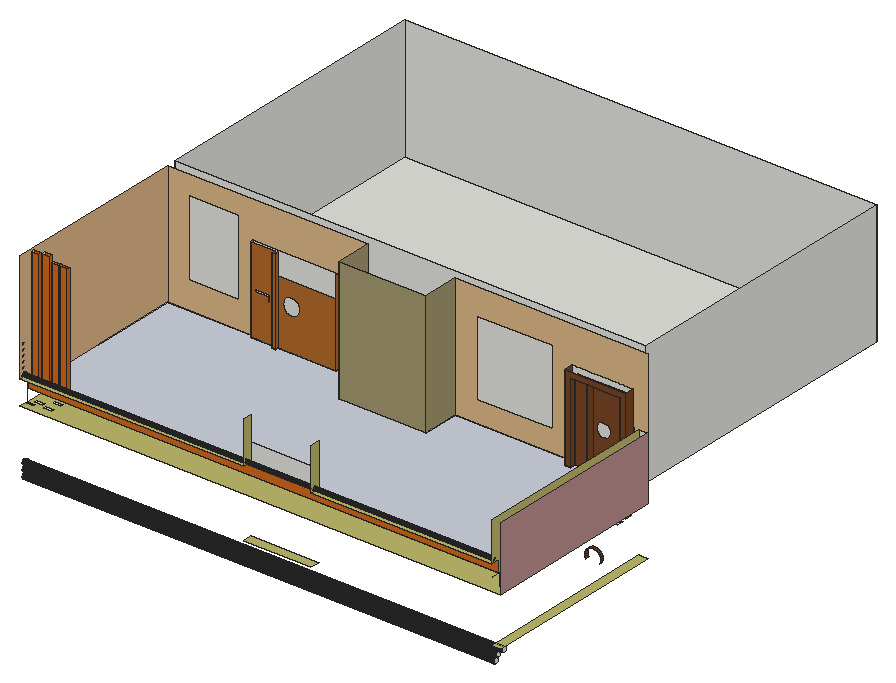
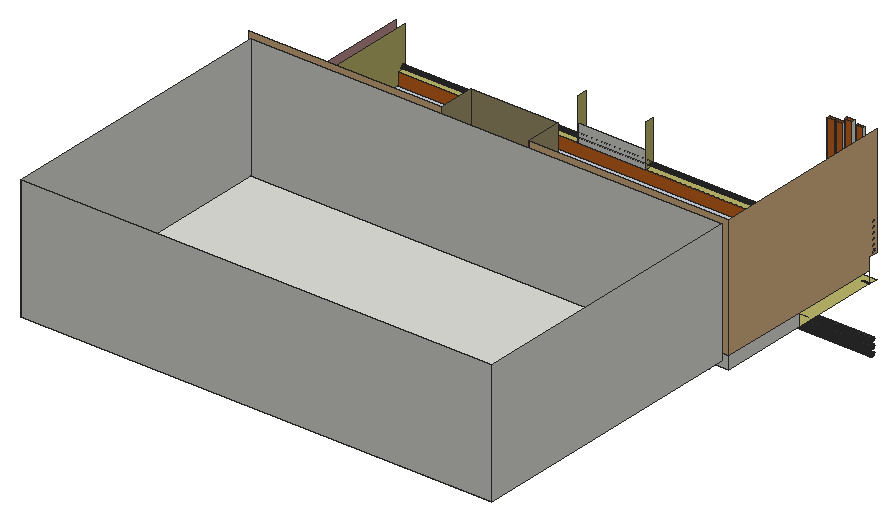
# SketchUp Ruby script. Lengths in inches.
U = 1.inch
M = Sketchup.active_model
def pt(a) = Geom::Point3d.new(a.map { |v| v * U })
def face(e, loops, mat)
  f = e.add_face(loops[0].map { |a| pt(a) })
  loops[1..].each { |l| e.add_face(l.map { |a| pt(a) }).erase! }
  f.material = f.back_material = mat if mat
  f
end
# faces: each face lists its corners as indices into pts; further lists are holes
def faces(e, pts, list, mat = nil) = list.each { |f| face(e, (f[0].is_a?(Array) ? f : [f]).map { |l| l.map { |i| pts[i] } }, mat) }
# xy, xz, yz: faces in a plane at the given z, y or x. An outline is a flat list of corners, or four numbers for a rectangle; further outlines are holes
def ring(l) = l.size == 4 ? [[l[0], l[1]], [l[2], l[1]], [l[2], l[3]], [l[0], l[3]]] : l.each_slice(2).to_a
def flat(e, list, mat, &to3) = list.each { |f| face(e, (f[0].is_a?(Array) ? f : [f]).map { |l| ring(l).map { |u, v| to3.(u, v) } }, mat) }
def xy(e, z, list, mat = nil) = flat(e, list, mat) { |x, y| [x, y, z] }
def xz(e, y, list, mat = nil) = flat(e, list, mat) { |x, z| [x, y, z] }
def yz(e, x, list, mat = nil) = flat(e, list, mat) { |y, z| [x, y, z] }
def lines(e, pts, list) = list.each { |a, b| e.add_line(pt(pts[a]), pt(pts[b])) }
# prism: a flat outline (further loops are holes) pulled along v
def prism(e, loops, v, mat = nil)
  f = face(e, loops, mat); d = Geom::Vector3d.new(v.map { |x| x * U })
  f.pushpull(f.normal.samedirection?(d) ? d.length : -d.length)
end
def box(e, o, s, mat = nil) = prism(e, [[o, [o[0] + s[0], o[1], o[2]], [o[0] + s[0], o[1] + s[1], o[2]], [o[0], o[1] + s[1], o[2]]]], [0, 0, s[2]], mat)
def at(x, y, z, deg = 0) = Geom::Transformation.translation(pt([x, y, z])) * Geom::Transformation.rotation(ORIGIN, Z_AXIS, deg.degrees)
def axes(o, x, y, z) = Geom::Transformation.new([*x, 0, *y, 0, *z, 0, *pt(o).to_a, 1])
def part(name) = M.definitions.add(name)
# library, detail: a bought-in or finely detailed component or shape, given as its bounding box
def library(name, o, s) = part(name).tap { |d| box(d.entities, o, s) }
def detail(e, o, s) = box(e.add_group.entities, o, s)
def put(e, d, t, mat = nil) = e.add_instance(d, t).tap { |i| i.material = mat if mat }
def group(e, t, mat = nil) = e.add_group.tap { |g| g.transformation = t; g.material = mat if mat }.entities
root = M.entities
M.materials.add("[0036_BurlyWood]").color = [222, 184, 135]
M.materials.add("[0041_Chocolate]").color = [210, 105, 30]
M.materials.add("[0057_DarkKhaki]").color = [189, 183, 107]
M.materials.add("[0119_RosyBrown]").color = [188, 143, 143]
M.materials.add("[Marble Carrara Floor Tile]").color = [204, 208, 219]
M.materials.add("[Sandstone]").color = [118, 81, 52]
M.materials.add("[Wood Bamboo]").color = [177, 105, 43]
M.materials.add("[Wood Floor Parquet]").color = [145, 89, 39]
M.materials.add("[Wood Lumber ButtJoined]").color = [164, 152, 112]
M.materials.add("[Wood Veneer 01]").color = [120, 70, 37]
xy(root,289,[[115.45,186.3,116.7,189.3]],"[Wood Bamboo]")
xy(root,292.0625,[[105.14,186.3,115.45,189.3]],"[Wood Bamboo]")
xy(root,293.5,[[105.14,186.3,116.7,189.3]],"[Wood Bamboo]")
xy(root,300,[[471,12,480,192.3]],"[0057_DarkKhaki]")
xy(root,306.625,[[227.54,12,293.97,21]],"[0057_DarkKhaki]")
xy(root,308.5,[[130.66,186.3,176.72,189.3]],"[Wood Bamboo]")
xy(root,320.5625,[[130.66,186.3,176.72,189.3]],"[Wood Bamboo]")
xy(root,324,[[395.16,186.3,410.94,189.3],[410.94,186.3,411.65,189.3],[411.65,186.3,455.16,189.3],[395.16,189.3,455.16,192.3]])
xy(root,324,[[120.23,186.3,123.15,189.3],[100.9,189.3,184.9,192.3]],"[Wood Bamboo]")
xy(root,331.9375,[[387.22,186.3,463.09,192.3]],"[Wood Veneer 01]")
xy(root,335.94,[[309.99,189.3,343.2,192.3],[347.01,189.3,376.42,192.3]])
xy(root,340.15,[[30.47,189.3,55.47,192.3],[60.04,189.3,80.47,192.3]],"[Wood Floor Parquet]")
xy(root,340.75,[[305.18,189.3,381.23,192.3]],"[Wood Floor Parquet]")
xy(root,344.59,[[26.03,189.3,84.9,192.3]],"[Wood Floor Parquet]")
xy(root,348,[[9,12,9,18.8125,16.75,18.8125,16.75,21,9,21,9,192.3,92.74,192.3,92.74,189.3,116.27,189.3,116.27,186.3,119.49,186.3,119.49,189.3,176.74,189.3,176.74,192.3,205.37,192.3,205.37,156.87,290.8125,156.87,290.8125,192.3,405.34,192.3,405.34,183.3,410.93,183.3,410.93,189.3,426.75,189.3,426.75,183.3,427.96,183.3,427.96,189.3,459.74,189.3,459.74,183.3,465.34,183.3,465.34,192.3,480,192.3,480,12]],"[0057_DarkKhaki]")
xy(root,349.8125,[[26.9375,18.8125,34.6875,21]])
xy(root,351.875,[[17.75,18.8125,25.5,21]])
xy(root,357.3125,[[35.9375,18.8125,43.6875,21]])
xy(root,360,[[471,21,471.0625,192.3],[405.34,183.3,410.93,192.3],[426.75,183.3,427.96,183.3,427.96,189.3,459.74,189.3,459.74,192.3,410.93,192.3,410.93,189.3,426.75,189.3],[459.74,183.3,465.34,192.3],[116.27,186.3,119.49,186.3,119.49,189.3,176.74,189.3,176.74,192.3,92.74,192.3,92.74,189.3,116.27,189.3],
  [9,201.23,471,483]])
xy(root,360,[[9,21,471,21,471,192.3,465.34,192.3,465.34,183.3,459.74,183.3,459.74,189.3,427.96,189.3,427.96,183.3,426.75,183.3,426.75,189.3,410.93,189.3,410.93,183.3,405.34,183.3,405.34,192.3,290.8125,192.3,290.8125,156.87,205.37,156.87,205.37,192.3,176.74,192.3,176.74,189.3,119.49,189.3,119.49,186.3,116.27,186.3,116.27,189.3,92.74,189.3,92.74,192.3,9,192.3]],"[Marble Carrara Floor Tile]")
xy(root,372,[[9,12,227.54,12,227.54,21,50.08,21,50.08,18,42.9,18,42.9,21,41.83,21,41.83,18,34.65,18,34.65,21,32.83,21,32.83,18,25.65,18,25.65,21,22.21,21,22.21,18,15.02,18,15.02,21,9,21],[293.97,12,471.0625,21]],"[0057_DarkKhaki]")
xz(root,18,[[15.02,372,22.21,483.12],[25.65,372,32.83,485],[34.65,372,41.83,479.9375],[42.9,372,50.08,480]],"[0041_Chocolate]")
xz(root,21,[[227.54,372,293.97,389.38]])
xz(root,21,[[9,360,9,372,15.02,372,15.02,483.12,22.21,483.12,22.21,372,25.65,372,25.65,485,32.83,485,32.83,372,34.65,372,34.65,479.9375,41.83,479.9375,41.83,372,42.9,372,42.9,480,50.08,480,50.08,372,471.0625,372,471.0625,360]],"[0041_Chocolate]")
xz(root,156.87,[[205.37,348,290.8125,360]])
xz(root,156.87,[[205.37,360,290.8125,480]],"[Wood Lumber ButtJoined]")
xz(root,183.3,[[405.34,348,410.93,360],[426.75,348,427.96,360],[459.74,348,465.34,360]])
xz(root,183.3,[[405.34,360,410.93,360,410.93,438.4,459.74,438.4,459.74,360,465.34,360,465.34,444,405.34,444],[426.75,360,427.96,438.4]],"[Wood Veneer 01]")
xz(root,186.3,[[116.27,348,119.49,360]])
xz(root,186.3,[[115.45,289,116.7,289,116.7,293.5,105.14,293.5,105.14,292.0625,115.45,292.0625],[130.66,308.5,176.72,320.5625],[116.27,360,119.49,444]],"[Wood Bamboo]")
xz(root,189.3,[[115.45,289,115.45,292.0625,105.14,292.0625,105.14,293.5,116.7,293.5,116.7,289],[130.66,308.5,176.72,320.5625],[92.74,348,116.27,360],[119.49,348,176.74,360],[410.93,348,426.75,360],
  [427.96,348,459.74,360]])
xz(root,189.3,[[[123.15,303.1875,184.9,324],[130.66,308.5,176.72,320.5625]],[[92.74,360,116.27,444],[109.64,396.16,109.64,401.1,96.64,401.1,96.64,403.6,111.7,403.6,111.7,396.16]],[[119.49,360,176.74,422.86],[132.85,392.25,130.72,392.53,128.73,393.36,127.02,394.67,125.71,396.38,124.88,398.37,124.6,400.5,124.88,402.64,125.71,404.63,127.02,406.34,128.73,407.65,130.72,408.47,132.85,408.75,134.99,408.47,136.98,407.65,138.68,406.34,140,404.63,140.82,402.64,141.1,400.5,140.82,398.37,140,396.38,138.68,394.67,136.98,393.36,134.99,392.53]]],"[Wood Bamboo]")
xz(root,189.3,[[410.93,360,426.75,438.4],[[427.96,360,459.74,438.4],[438.92,392.76,437.13,393,435.46,393.69,434.02,394.8,432.92,396.23,432.22,397.91,431.99,399.7,432.22,401.5,432.92,403.17,434.02,404.61,435.46,405.71,437.13,406.4,438.92,406.64,440.72,406.4,442.39,405.71,443.83,404.61,444.93,403.17,445.625,401.5,445.86,399.7,445.625,397.91,444.93,396.23,443.83,394.8,442.39,393.69,440.72,393]]],"[Wood Veneer 01]")
xz(root,192.3,[[9,348,92.74,360],[176.74,348,205.37,360],[290.8125,348,405.34,360],[465.34,348,466.21,360],[466.21,348,471,360],
  [471,348,480,360],[405.34,360,405.34,444,465.34,444,465.34,360,459.74,360,459.74,438.4,410.93,438.4,410.93,360],[471.0625,360,480,396]])
xz(root,192.3,[[[9,360,92.74,360,92.74,444,176.74,444,176.74,360,205.37,360,205.37,480,9,480],[29.8125,386.98,79,461.6]],[[290.8125,360,405.34,360,405.34,444,465.34,444,465.34,360,471.0625,360,471.0625,410.4375,480,410.4375,480,480,290.8125,480],[312.25,380.84,386.1875,454.78]]],"[0036_BurlyWood]")
xz(root,201.23,[[9,360,471,480]])
xz(root,483,[[9,360,471,480]])
yz(root,9,[[106.65,348,192.3,360],[201.23,360,483,480],[15.36,372.95,14.91,373.01,14.49,373.1875,14.125,373.47,13.85,373.83,13.67,374.25,13.61,374.7,13.67,375.16,13.85,375.58,14.125,375.94,14.49,376.22,14.91,376.39,15.36,376.45,15.82,376.39,16.24,376.22,16.6,375.94,16.88,375.58,17.05,375.16,17.11,374.7,17.05,374.25,16.88,373.83,16.6,373.47,16.24,373.1875,15.82,373.01]])
yz(root,9,[[[21,360,192.3,360,192.3,480,12,480,12,372,21,372],[15.36,399.52,14.91,399.58,14.49,399.75,14.125,400.03,13.85,400.39,13.67,400.8125,13.61,401.27,13.67,401.72,13.85,402.14,14.125,402.5,14.49,402.78,14.91,402.96,15.36,403.02,15.82,402.96,16.24,402.78,16.6,402.5,16.88,402.14,17.05,401.72,17.11,401.27,17.05,400.8125,16.88,400.39,16.6,400.03,16.24,399.75,15.82,399.58],[15.36,394.2,14.91,394.26,14.49,394.4375,14.125,394.72,13.85,395.08,13.67,395.5,13.61,395.95,13.67,396.41,13.85,396.83,14.125,397.19,14.49,397.47,14.91,397.64,15.36,397.7,15.82,397.64,16.24,397.47,16.6,397.19,16.88,396.83,17.05,396.41,17.11,395.95,17.05,395.5,16.88,395.08,16.6,394.72,16.24,394.4375,15.82,394.26],[15.36,388.89,14.91,388.95,14.49,389.125,14.125,389.4,13.85,389.77,13.67,390.1875,13.61,390.64,13.67,391.09,13.85,391.52,14.125,391.88,14.49,392.16,14.91,392.33,15.36,392.39,15.82,392.33,16.24,392.16,16.6,391.88,16.88,391.52,17.05,391.09,17.11,390.64,17.05,390.1875,16.88,389.77,16.6,389.4,16.24,389.125,15.82,388.95],[15.36,383.58,14.91,383.64,14.49,383.8125,14.125,384.09,13.85,384.45,13.67,384.875,13.61,385.33,13.67,385.78,13.85,386.2,14.125,386.57,14.49,386.84,14.91,387.02,15.36,387.08,15.82,387.02,16.24,386.84,16.6,386.57,16.88,386.2,17.05,385.78,17.11,385.33,17.05,384.875,16.88,384.45,16.6,384.09,16.24,383.8125,15.82,383.64],[15.36,378.27,14.91,378.33,14.49,378.5,14.125,378.78,13.85,379.14,13.67,379.5625,13.61,380.02,13.67,380.47,13.85,380.89,14.125,381.25,14.49,381.53,14.91,381.71,15.36,381.77,15.82,381.71,16.24,381.53,16.6,381.25,16.88,380.89,17.05,380.47,17.11,380.02,17.05,379.5625,16.88,379.14,16.6,378.78,16.24,378.5,15.82,378.33],[15.36,372.95,14.91,373.01,14.49,373.1875,14.125,373.47,13.85,373.83,13.67,374.25,13.61,374.7,13.67,375.16,13.85,375.58,14.125,375.94,14.49,376.22,14.91,376.39,15.36,376.45,15.82,376.39,16.24,376.22,16.6,375.94,16.88,375.58,17.05,375.16,17.11,374.7,17.05,374.25,16.88,373.83,16.6,373.47,16.24,373.1875,15.82,373.01]]],"[0036_BurlyWood]")
yz(root,15.02,[[18,372,21,483.12]])
yz(root,22.21,[[18,372,21,483.12]],"[0041_Chocolate]")
yz(root,25.65,[[18,372,21,485]])
yz(root,32.83,[[18,372,21,485]],"[0041_Chocolate]")
yz(root,34.65,[[18,372,21,479.9375]])
yz(root,41.83,[[18,372,21,479.9375]],"[0041_Chocolate]")
yz(root,42.9,[[18,372,21,480]])
yz(root,50.08,[[18,372,21,480]],"[0041_Chocolate]")
yz(root,92.74,[[189.3,348,192.3,360]])
yz(root,92.74,[[189.3,360,192.3,444]],"[Wood Bamboo]")
yz(root,105.14,[[186.3,292.0625,189.3,293.5]],"[Wood Bamboo]")
yz(root,115.45,[[186.3,289,189.3,292.0625]],"[Wood Bamboo]")
yz(root,116.27,[[186.3,348,189.3,360]])
yz(root,116.27,[[186.3,360,189.3,444]],"[Wood Bamboo]")
yz(root,116.7,[[186.3,289,189.3,293.5]],"[Wood Bamboo]")
yz(root,119.49,[[186.3,348,189.3,360]])
yz(root,119.49,[[186.3,360,189.3,444]],"[Wood Bamboo]")
yz(root,130.66,[[186.3,308.5,189.3,320.5625]],"[Wood Bamboo]")
yz(root,176.72,[[186.3,308.5,189.3,320.5625]],"[Wood Bamboo]")
yz(root,176.74,[[189.3,348,192.3,360]])
yz(root,176.74,[[189.3,360,192.3,444]],"[Wood Bamboo]")
yz(root,205.37,[[156.87,348,192.3,360]])
yz(root,205.37,[[156.87,360,192.3,480]],"[Wood Lumber ButtJoined]")
yz(root,227.54,[[12,372,21,413.38]],"[0057_DarkKhaki]")
yz(root,290.8125,[[156.87,348,192.3,360]])
yz(root,290.8125,[[156.87,360,192.3,480]],"[Wood Lumber ButtJoined]")
yz(root,293.97,[[12,372,21,413.38]],"[0057_DarkKhaki]")
yz(root,405.34,[[183.3,348,192.3,360]])
yz(root,405.34,[[183.3,360,192.3,444]],"[Wood Veneer 01]")
yz(root,410.93,[[183.3,348,189.3,360],[189.3,360,192.3,438.4]])
yz(root,410.93,[[183.3,360,189.3,438.4]],"[Wood Veneer 01]")
yz(root,426.75,[[183.3,348,189.3,360]])
yz(root,426.75,[[183.3,360,189.3,438.4]],"[Wood Veneer 01]")
yz(root,427.96,[[183.3,348,189.3,360]])
yz(root,427.96,[[183.3,360,189.3,438.4]],"[Wood Veneer 01]")
yz(root,459.74,[[183.3,348,189.3,360],[189.3,360,192.3,438.4]])
yz(root,459.74,[[183.3,360,189.3,438.4]],"[Wood Veneer 01]")
yz(root,465.34,[[183.3,348,192.3,360]])
yz(root,465.34,[[183.3,360,192.3,444]],"[Wood Veneer 01]")
yz(root,471,[[201.23,360,483,480]])
yz(root,471.0625,[[[21,360,21,372,12,372,12,410.4375,192.3,410.4375,192.3,360],[15.36,372.95,15.82,373.01,16.24,373.1875,16.6,373.47,16.88,373.83,17.05,374.25,17.11,374.7,17.05,375.16,16.88,375.58,16.6,375.94,16.24,376.22,15.82,376.39,15.36,376.45,14.91,376.39,14.49,376.22,14.125,375.94,13.85,375.58,13.67,375.16,13.61,374.7,13.67,374.25,13.85,373.83,14.125,373.47,14.49,373.1875,14.91,373.01]]],"[0057_DarkKhaki]")
yz(root,471.75,[[16.59,282.52,17.16,282.6,17.69,282.82,18.14,283.16,18.49,283.62,18.7,284.15,18.78,284.71,18.7,285.28,18.49,285.81,18.14,286.26,17.69,286.61,17.16,286.82,16.59,286.9,16.03,286.82,15.5,286.61,15.04,286.26,14.7,285.81,14.48,285.28,14.4,284.71,14.48,284.15,14.7,283.62,15.04,283.16,15.5,282.82,16.03,282.6]])
yz(root,473.625,[[16.59,288.9,17.16,288.97,17.69,289.19,18.14,289.54,18.49,289.99,18.7,290.52,18.78,291.09,18.7,291.65,18.49,292.18,18.14,292.63,17.69,292.98,17.16,293.2,16.59,293.27,16.03,293.2,15.5,292.98,15.04,292.63,14.7,292.18,14.48,291.65,14.4,291.09,14.48,290.52,14.7,289.99,15.04,289.54,15.5,289.19,16.03,288.97]])
yz(root,479.625,[[16.59,295.27,17.16,295.35,17.69,295.57,18.14,295.91,18.49,296.37,18.7,296.9,18.78,297.46,18.7,298.03,18.49,298.56,18.14,299.01,17.69,299.36,17.16,299.57,16.59,299.65,16.03,299.57,15.5,299.36,15.04,299.01,14.7,298.56,14.48,298.03,14.4,297.46,14.48,296.9,14.7,296.37,15.04,295.91,15.5,295.57,16.03,295.35]])
yz(root,480,[[12,348,192.3,410.4375]],"[0119_RosyBrown]")
p = [[9,16.03,282.6],[9,16.59,282.52],[471.75,16.59,282.52],[471.75,16.03,282.6],[9,17.16,282.6],[471.75,17.16,282.6],
  [9,15.5,282.82],[471.75,15.5,282.82],[9,17.69,282.82],[471.75,17.69,282.82],[9,15.04,283.16],[471.75,15.04,283.16],
  [9,18.14,283.16],[471.75,18.14,283.16],[423.06,189.3,284.87],[423.83,189.3,283],[423.83,186.3,283],[423.06,186.3,284.87],
  [437.26,189.3,283],[438.03,189.3,284.87],[438.03,186.3,284.87],[437.26,186.3,283],[9,14.7,283.62],[471.75,14.7,283.62],
  [9,18.49,283.62],[471.75,18.49,283.62],[9,14.48,284.15],[471.75,14.48,284.15],[9,18.7,284.15],[471.75,18.7,284.15],
  [137.79,189.3,286.34],[135.49,189.3,283.8125],[135.49,186.3,283.8125],[137.79,186.3,286.34],[9,14.4,284.71],[471.75,14.4,284.71],
  [9,18.78,284.71],[471.75,18.78,284.71],[9,14.48,285.28],[471.75,14.48,285.28],[9,18.7,285.28],[471.75,18.7,285.28],
  [156.19,189.3,284.8],[153.67,189.3,287.09],[153.67,186.3,287.09],[156.19,186.3,284.8],[422.79,189.3,286.88],[422.79,186.3,286.88],
  [438.29,189.3,286.88],[438.29,186.3,286.88],[9,14.7,285.81],[471.75,14.7,285.81],[9,18.49,285.81],[471.75,18.49,285.81],
  [9,15.04,286.26],[471.75,15.04,286.26],[9,18.14,286.26],[471.75,18.14,286.26],[9,15.5,286.61],[471.75,15.5,286.61],
  [9,17.69,286.61],[471.75,17.69,286.61],[140.65,189.3,288.18],[140.65,186.3,288.18],[9,16.03,286.82],[471.75,16.03,286.82],
  [9,17.16,286.82],[471.75,17.16,286.82],[9,16.59,286.9],[471.75,16.59,286.9],[423.06,189.3,288.88],[423.06,186.3,288.88],
  [438.03,189.3,288.88],[438.03,186.3,288.88],[150.64,189.3,288.66],[150.64,186.3,288.66],[143.9,189.3,289.22],[143.9,186.3,289.22],
  [147.31,189.3,289.38],[147.31,186.3,289.38],[9,16.03,288.97],[9,16.59,288.9],[473.625,16.59,288.9],[473.625,16.03,288.97],
  [9,17.16,288.97],[473.625,17.16,288.97],[423.83,189.3,290.75],[423.83,186.3,290.75],[437.26,189.3,290.75],[437.26,186.3,290.75],
  [9,15.5,289.19],[473.625,15.5,289.19],[9,17.69,289.19],[473.625,17.69,289.19],[9,15.04,289.54],[473.625,15.04,289.54],
  [9,18.14,289.54],[473.625,18.14,289.54],[9,14.7,289.99],[473.625,14.7,289.99],[9,18.49,289.99],[473.625,18.49,289.99],
  [9,14.48,290.52],[473.625,14.48,290.52],[9,18.7,290.52],[473.625,18.7,290.52],[9,14.4,291.09],[473.625,14.4,291.09],
  [9,18.78,291.09],[473.625,18.78,291.09],[425.0625,189.3,292.36],[425.0625,186.3,292.36],[436.02,189.3,292.36],[436.02,186.3,292.36],
  [9,14.48,291.65],[473.625,14.48,291.65],[9,18.7,291.65],[473.625,18.7,291.65],[9,14.7,292.18],[473.625,14.7,292.18],
  [9,18.49,292.18],[473.625,18.49,292.18],[9,15.04,292.63],[473.625,15.04,292.63],[9,18.14,292.63],[473.625,18.14,292.63],
  [426.67,189.3,293.59],[426.67,186.3,293.59],[434.42,189.3,293.59],[434.42,186.3,293.59],[9,15.5,292.98],[473.625,15.5,292.98],
  [9,17.69,292.98],[473.625,17.69,292.98],[9,16.03,293.2],[473.625,16.03,293.2],[9,17.16,293.2],[473.625,17.16,293.2],
  [9,16.59,293.27],[473.625,16.59,293.27],[428.54,189.3,294.36],[428.54,186.3,294.36],[432.55,189.3,294.36],[432.55,186.3,294.36],
  [430.54,189.3,294.63],[430.54,186.3,294.63],[9,15.5,295.57],[9,16.03,295.35],[479.625,16.03,295.35],[479.625,15.5,295.57],
  [9,16.59,295.27],[479.625,16.59,295.27],[9,17.16,295.35],[479.625,17.16,295.35],[9,17.69,295.57],[479.625,17.69,295.57],
  [9,15.04,295.91],[479.625,15.04,295.91],[9,18.14,295.91],[479.625,18.14,295.91],[9,14.7,296.37],[479.625,14.7,296.37],
  [9,18.49,296.37],[479.625,18.49,296.37],[9,14.48,296.9],[479.625,14.48,296.9],[9,18.7,296.9],[479.625,18.7,296.9],
  [9,14.4,297.46],[479.625,14.4,297.46],[9,18.78,297.46],[479.625,18.78,297.46],[9,14.48,298.03],[479.625,14.48,298.03],
  [9,18.7,298.03],[479.625,18.7,298.03],[9,14.7,298.56],[479.625,14.7,298.56],[9,18.49,298.56],[479.625,18.49,298.56],
  [9,15.04,299.01],[479.625,15.04,299.01],[9,18.14,299.01],[479.625,18.14,299.01],[9,15.5,299.36],[479.625,15.5,299.36],
  [9,17.69,299.36],[479.625,17.69,299.36],[9,16.03,299.57],[479.625,16.03,299.57],[9,17.16,299.57],[479.625,17.16,299.57],
  [9,16.59,299.65],[479.625,16.59,299.65],[9,14.49,373.1875],[9,14.91,373.01],[471.0625,14.91,373.01],[471.0625,14.49,373.1875],
  [9,15.36,372.95],[471.0625,15.36,372.95],[9,15.82,373.01],[471.0625,15.82,373.01],[9,16.24,373.1875],[471.0625,16.24,373.1875],
  [9,14.125,373.47],[471.0625,14.125,373.47],[9,16.6,373.47],[471.0625,16.6,373.47],[9,13.85,373.83],[471.0625,13.85,373.83],
  [9,16.88,373.83],[471.0625,16.88,373.83],[9,13.67,374.25],[471.0625,13.67,374.25],[9,17.05,374.25],[471.0625,17.05,374.25],
  [9,13.61,374.7],[471.0625,13.61,374.7],[9,17.11,374.7],[471.0625,17.11,374.7],[9,13.67,375.16],[471.0625,13.67,375.16],
  [9,17.05,375.16],[471.0625,17.05,375.16],[9,13.85,375.58],[471.0625,13.85,375.58],[9,16.88,375.58],[471.0625,16.88,375.58],
  [9,14.125,375.94],[471.0625,14.125,375.94],[9,16.6,375.94],[471.0625,16.6,375.94],[9,14.49,376.22],[471.0625,14.49,376.22],
  [9,16.24,376.22],[471.0625,16.24,376.22],[9,14.91,376.39],[471.0625,14.91,376.39],[9,15.82,376.39],[471.0625,15.82,376.39],
  [9,15.36,376.45],[471.0625,15.36,376.45],[9,106.65,360],[0,106.65,360],[471,201.23,360],[471,192.3,360],
  [9,21,360],[9,21,348],[471,21,360],[471,21,348],[471.0625,21,360],[471.0625,12,360],
  [466.21,192.3,360],[466.21,192.3,410.4375]]
faces(root,p,[[0,1,2,3],[1,4,5,2],[6,0,3,7],[4,8,9,5],[10,6,7,11],[8,12,13,9],[22,10,11,23],[12,24,25,13],
  [26,22,23,27],[24,28,29,25],[34,26,27,35],[28,36,37,29],[38,34,35,39],[36,40,41,37],[50,38,39,51],[40,52,53,41],
  [54,50,51,55],[52,56,57,53],[58,54,55,59],[56,60,61,57],[64,58,59,65],[60,66,67,61],[68,64,65,69],[66,68,69,67],
  [80,81,82,83],[81,84,85,82],[90,80,83,91],[84,92,93,85],[94,90,91,95],[92,96,97,93],[98,94,95,99],[96,100,101,97],
  [102,98,99,103],[100,104,105,101],[106,102,103,107],[104,108,109,105],[114,106,107,115],[108,116,117,109],[118,114,115,119],[116,120,121,117],
  [122,118,119,123],[120,124,125,121],[130,122,123,131],[124,132,133,125],[134,130,131,135],[132,136,137,133],[138,134,135,139],[136,138,139,137],
  [146,147,148,149],[147,150,151,148],[150,152,153,151],[152,154,155,153],[156,146,149,157],[154,158,159,155],[160,156,157,161],[158,162,163,159],
  [164,160,161,165],[162,166,167,163],[168,164,165,169],[166,170,171,167],[172,168,169,173],[170,174,175,171],[176,172,173,177],[174,178,179,175],
  [180,176,177,181],[178,182,183,179],[184,180,181,185],[182,186,187,183],[188,184,185,189],[186,190,191,187],[192,188,189,193],[190,192,193,191],
  [194,195,196,197],[195,198,199,196],[198,200,201,199],[200,202,203,201],[204,194,197,205],[202,206,207,203],[208,204,205,209],[206,210,211,207],
  [212,208,209,213],[210,214,215,211],[216,212,213,217],[214,218,219,215],[220,216,217,221],[218,222,223,219],[224,220,221,225],[222,226,227,223],
  [228,224,225,229],[226,230,231,227],[232,228,229,233],[230,234,235,231],[236,232,233,237],[234,238,239,235],[240,236,237,241],[238,240,241,239]],"[Sandstone]")
faces(root,p,[[14,15,16,17],[18,19,20,21],[46,14,17,47],[19,48,49,20],[70,46,47,71],[48,72,73,49],[86,70,71,87],[72,88,89,73],
  [110,86,87,111],[88,112,113,89],[126,110,111,127],[112,128,129,113],[140,126,127,141],[128,142,143,129],[144,140,141,145],[142,144,145,143]],"[Wood Veneer 01]")
faces(root,p,[[30,31,32,33],[42,43,44,45],[62,30,33,63],[43,74,75,44],[76,62,63,77],[74,78,79,75],[78,76,77,79]],"[Wood Bamboo]")
lines(root,p,[[242,243],[244,245],[246,247],[248,249],[250,251],[252,253]])
